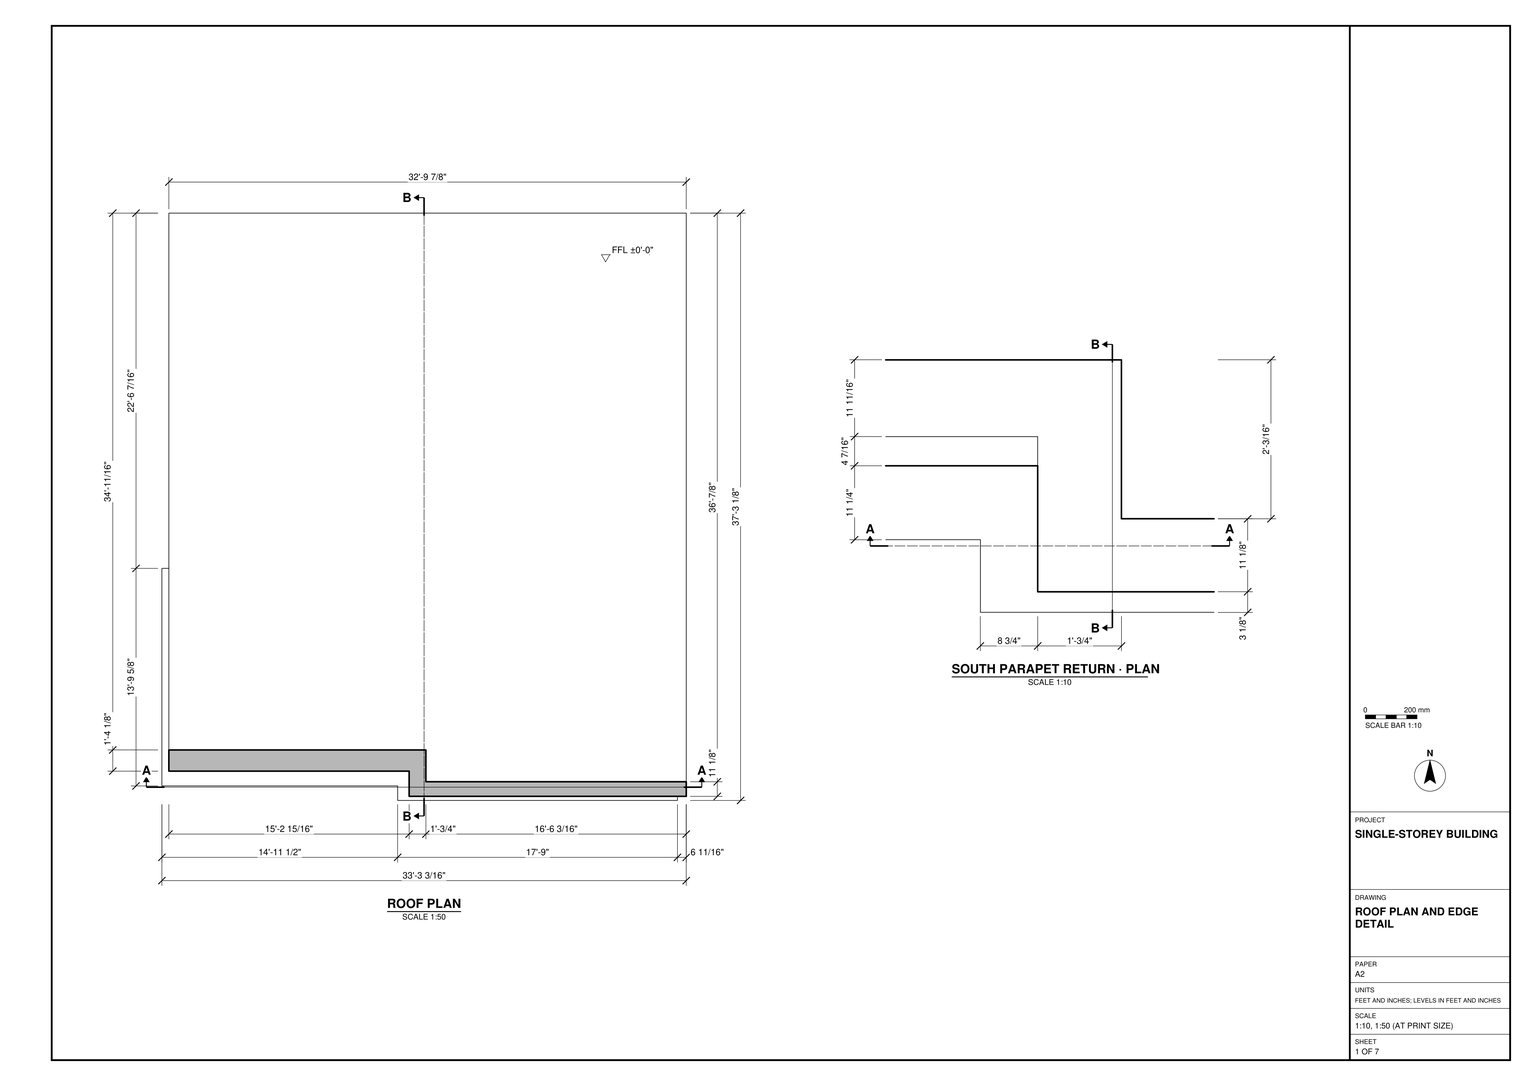
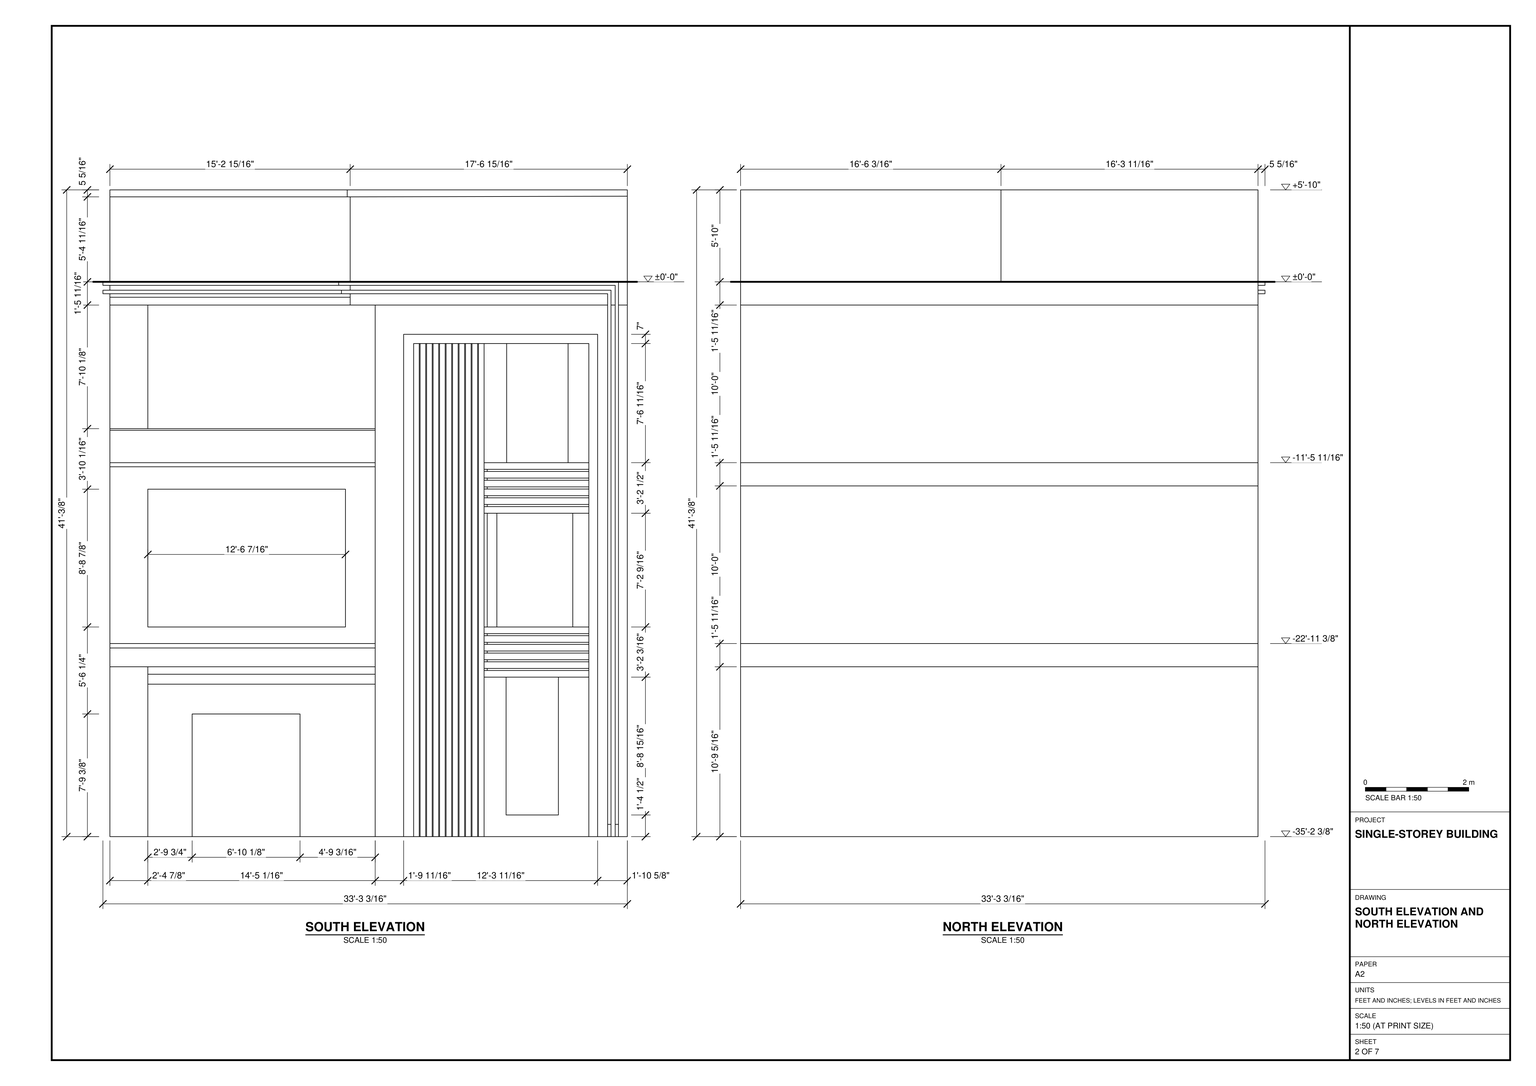
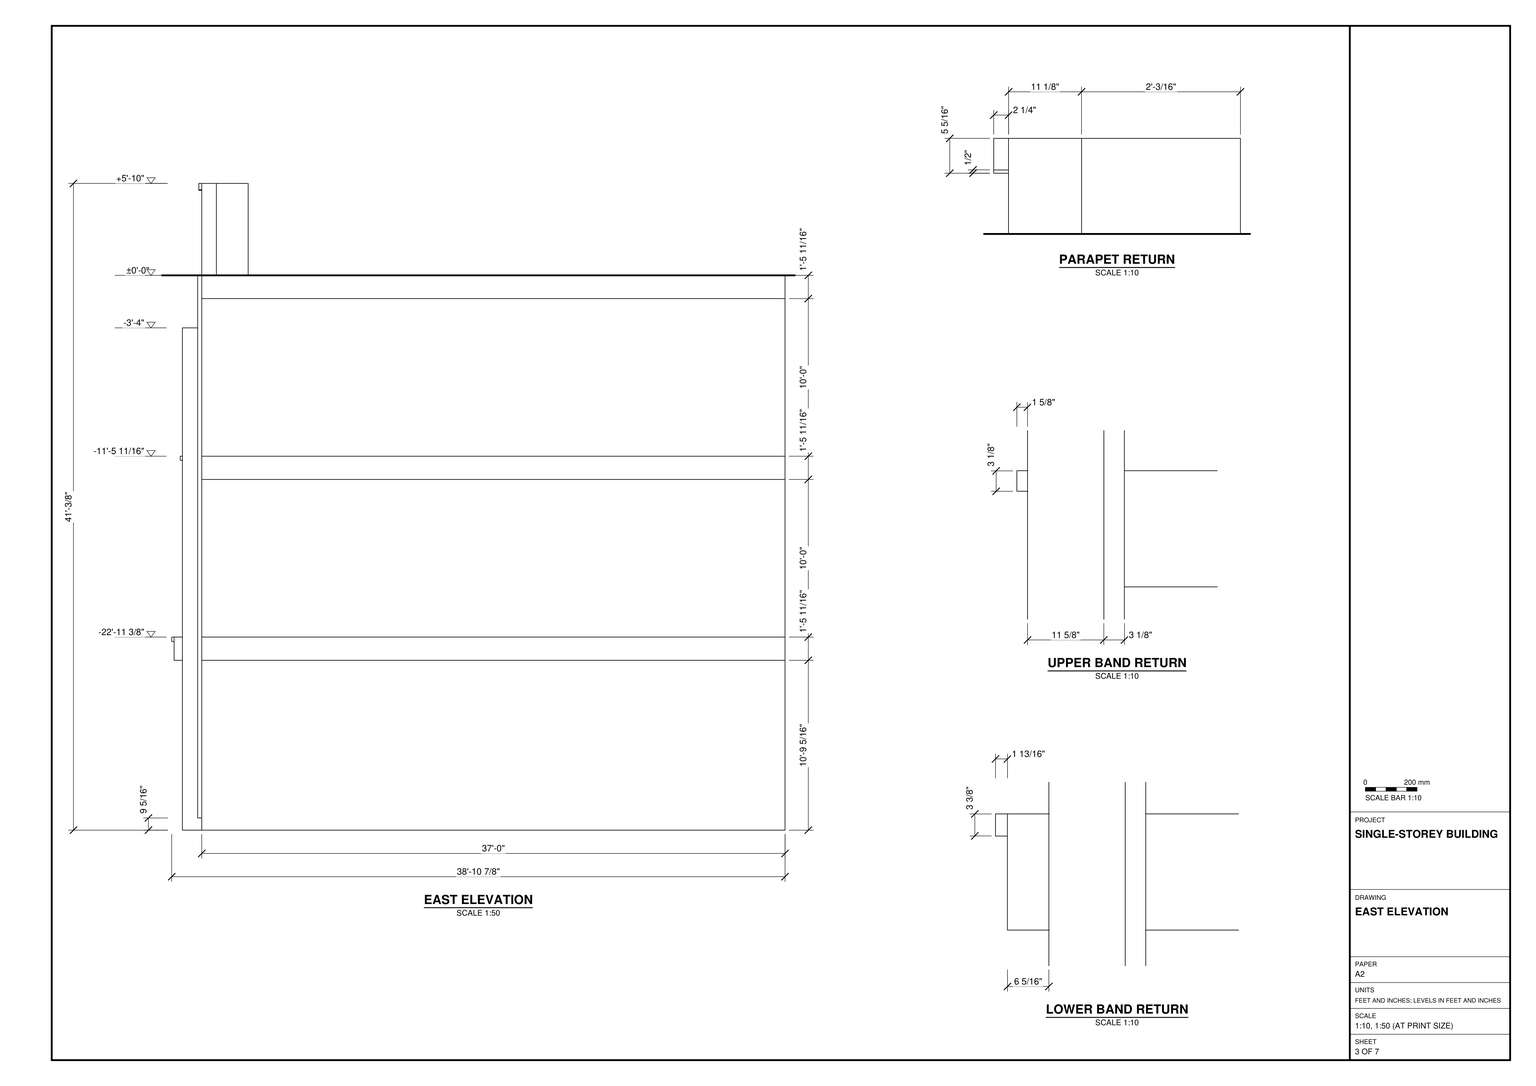
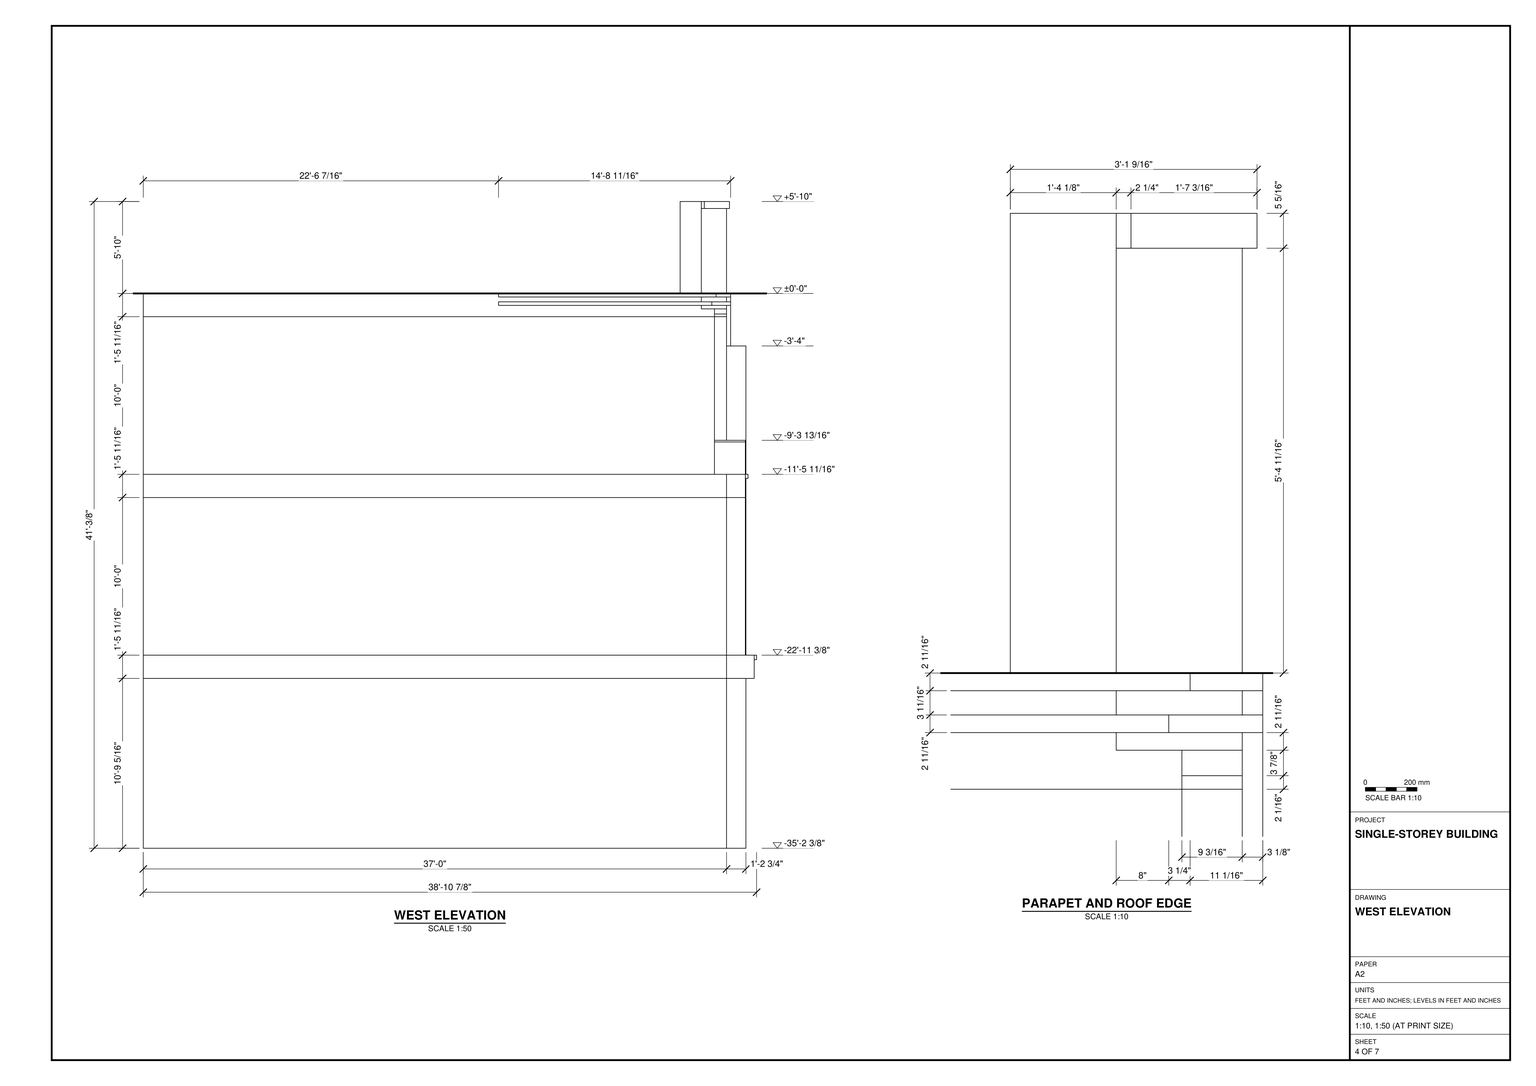
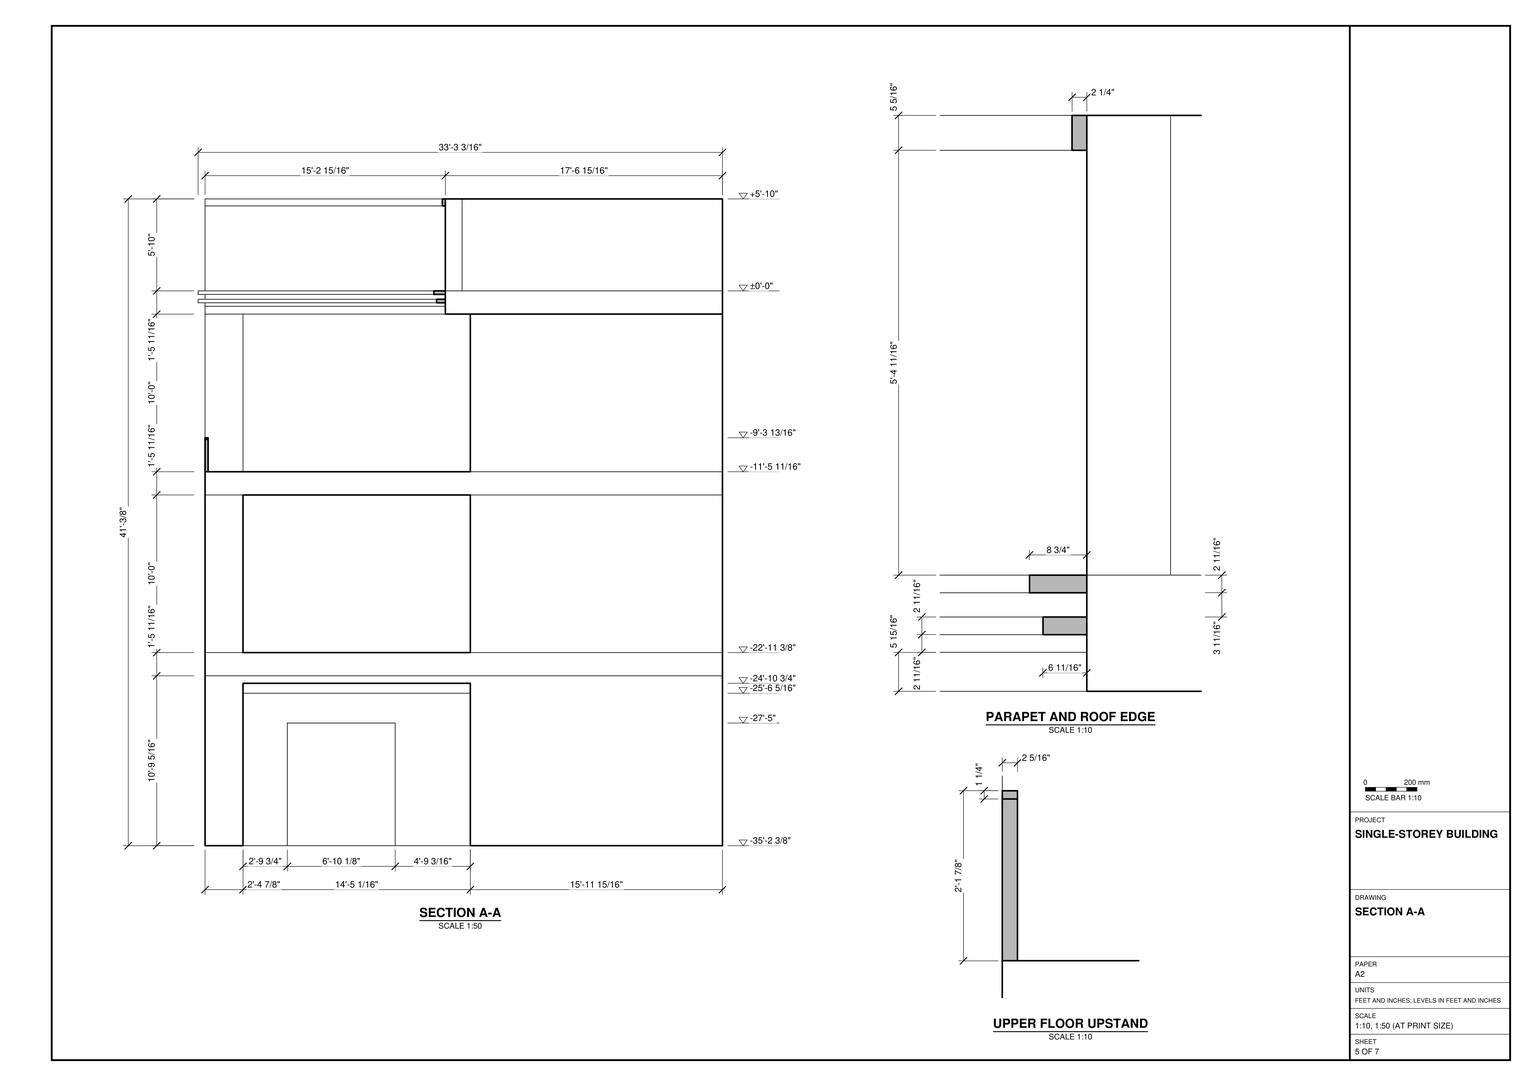
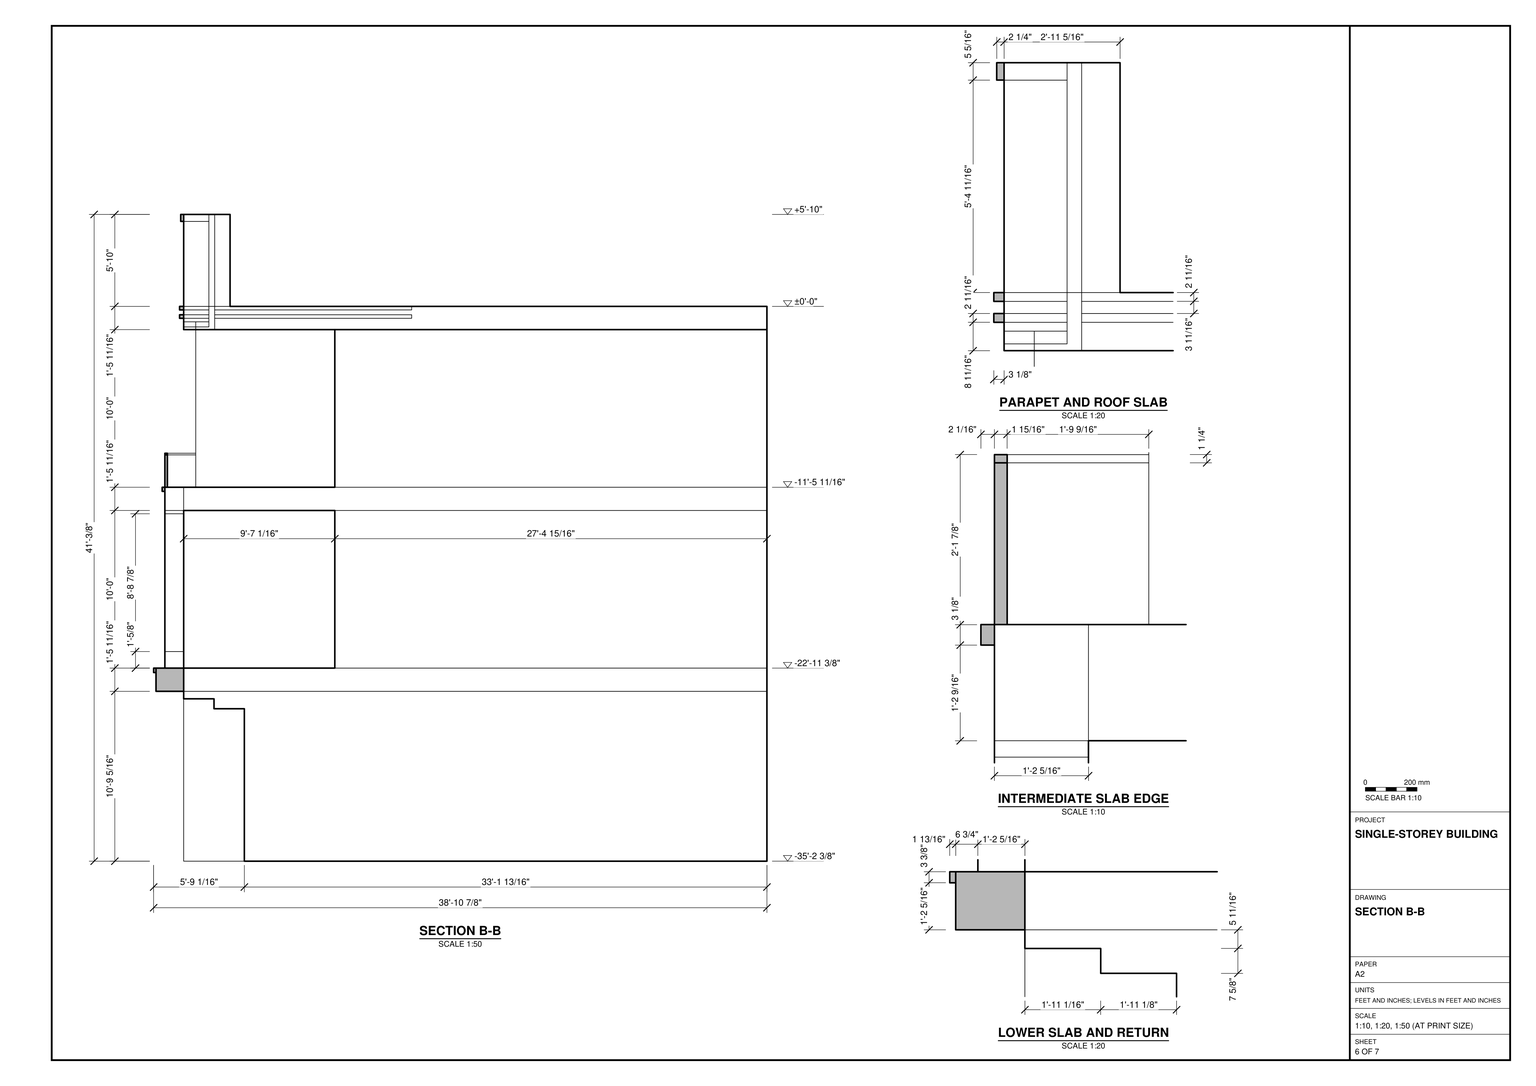
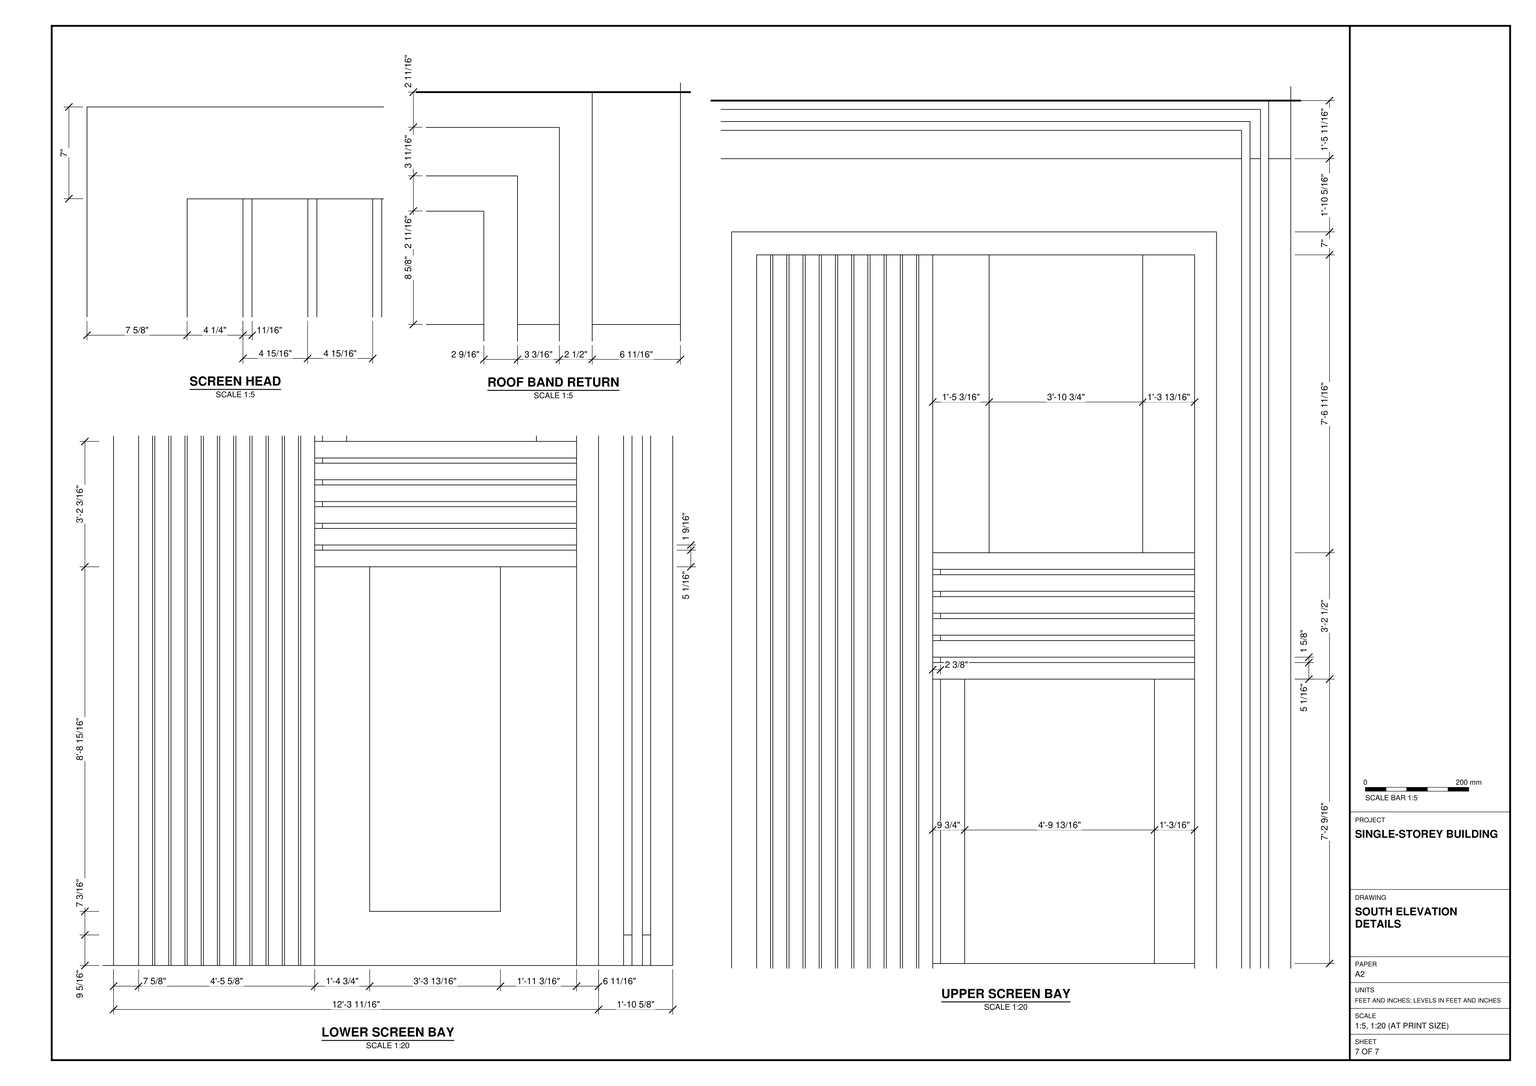
Build the exterior shell in SketchUp from task_files/diagram_01.pdf. Work in feet and inches. The overall dimensions, including projections, are 33'-3 3/16" east to west, 38'-10 7/8" north to south and 41'-3/8" high. Use the marked level ±0'-0" at the roof plane; the main wall faces extend below this datum and the south parapet rises above it.

Set out the walls and flat roof slab with the thicknesses shown. Follow the roof plan at the south edge, where a short return connects the two offset lengths of parapet. Use the elevations to align the slab edges and horizontal bands. On the south face, distinguish the broad left bay with its rectangular openings from the tall framed bay on the right. Within the frame, run the vertical fins alongside the stacked panels and horizontal slats. Use the edge details to give the bands, frame and parapet their drawn projections rather than representing them only with lines on a flat face.

Keep walls, slabs, roof and any furniture or joinery pieces shown in separate groups or components, and use components for repeated parts such as the fins. Any decor or loose items shown may use suitable library components. Save one SketchUp model as output_files/building_shell_with_stepped_parapet_and_screened_facade.skp.

# SketchUp Ruby script. Lengths in inches.
U = 1.inch
M = Sketchup.active_model
def pt(a) = Geom::Point3d.new(a.map { |v| v * U })
def face(e, loops, mat)
  f = e.add_face(loops[0].map { |a| pt(a) })
  loops[1..].each { |l| e.add_face(l.map { |a| pt(a) }).erase! }
  f.material = f.back_material = mat if mat
  f
end
# faces: each face lists its corners as indices into pts; further lists are holes
def faces(e, pts, list, mat = nil) = list.each { |f| face(e, (f[0].is_a?(Array) ? f : [f]).map { |l| l.map { |i| pts[i] } }, mat) }
# xy, xz, yz: faces in a plane at the given z, y or x. An outline is a flat list of corners, or four numbers for a rectangle; further outlines are holes
def ring(l) = l.size == 4 ? [[l[0], l[1]], [l[2], l[1]], [l[2], l[3]], [l[0], l[3]]] : l.each_slice(2).to_a
def flat(e, list, mat, &to3) = list.each { |f| face(e, (f[0].is_a?(Array) ? f : [f]).map { |l| ring(l).map { |u, v| to3.(u, v) } }, mat) }
def xy(e, z, list, mat = nil) = flat(e, list, mat) { |x, y| [x, y, z] }
def xz(e, y, list, mat = nil) = flat(e, list, mat) { |x, z| [x, y, z] }
def yz(e, x, list, mat = nil) = flat(e, list, mat) { |y, z| [x, y, z] }
def lines(e, pts, list) = list.each { |a, b| e.add_line(pt(pts[a]), pt(pts[b])) }
# prism: a flat outline (further loops are holes) pulled along v
def prism(e, loops, v, mat = nil)
  f = face(e, loops, mat); d = Geom::Vector3d.new(v.map { |x| x * U })
  f.pushpull(f.normal.samedirection?(d) ? d.length : -d.length)
end
def box(e, o, s, mat = nil) = prism(e, [[o, [o[0] + s[0], o[1], o[2]], [o[0] + s[0], o[1] + s[1], o[2]], [o[0], o[1] + s[1], o[2]]]], [0, 0, s[2]], mat)
def at(x, y, z, deg = 0) = Geom::Transformation.translation(pt([x, y, z])) * Geom::Transformation.rotation(ORIGIN, Z_AXIS, deg.degrees)
def axes(o, x, y, z) = Geom::Transformation.new([*x, 0, *y, 0, *z, 0, *pt(o).to_a, 1])
def part(name) = M.definitions.add(name)
# library, detail: a bought-in or finely detailed component or shape, given as its bounding box
def library(name, o, s) = part(name).tap { |d| box(d.entities, o, s) }
def detail(e, o, s) = box(e.add_group.entities, o, s)
def put(e, d, t, mat = nil) = e.add_instance(d, t).tap { |i| i.material = mat if mat }
def group(e, t, mat = nil) = e.add_group.tap { |g| g.transformation = t; g.material = mat if mat }.entities
root = M.entities
xy(root,-9.3125,[[228.91,8.125,228.91,22.875,207.25,22.875,207.25,69.0625,34.1875,69.0625,34.1875,22.875,5.3125,22.875,5.3125,466.875,399.1875,466.875,399.1875,22.875,376.59,22.875,376.59,8.125,369.9,8.125,369.9,22.875,290.16,22.875,290.16,18.625,285.91,18.625,285.91,22.875,285.22,22.875,285.22,18.625,280.97,18.625,280.97,22.875,280.29,22.875,280.29,18.625,276.04,18.625,276.04,22.875,275.35,22.875,275.35,18.625,271.1,18.625,271.1,22.875,270.41,22.875,270.41,18.625,266.16,18.625,266.16,22.875,265.47,22.875,265.47,18.625,261.22,18.625,261.22,22.875,260.54,22.875,260.54,18.625,256.29,18.625,256.29,22.875,255.6,22.875,255.6,18.625,251.35,18.625,251.35,22.875,250.66,22.875,250.66,18.625,246.41,18.625,246.41,22.875,245.72,22.875,245.72,18.625,241.47,18.625,241.47,22.875,240.79,22.875,240.79,18.625,236.54,18.625,236.54,8.125]])
xy(root,0,[[384.22,19.75,386.78,22.875],[389.97,19.75,392.47,22.875]])
xy(root,106.75,[[34.1875,45.97,207.25,69.0625]])
xy(root,112.11,[[290.16,16.125,369.9,22.875]])
xy(root,114.3125,[[34.1875,22.875,207.25,45.97]])
xy(root,117.17,[[290.16,16.125,369.9,22.875]])
xy(root,118.74,[[290.16,16.125,369.9,22.875]])
xy(root,120,[[5.3125,1.8125,34.1875,22.875],[34.1875,1.8125,207.25,22.875]])
xy(root,123.79,[[290.16,16.125,369.9,22.875]])
xy(root,125.36,[[290.16,16.125,369.9,22.875]])
xy(root,130.42,[[290.16,16.125,369.9,22.875]])
xy(root,131.99,[[290.16,16.125,369.9,22.875]])
xy(root,134.3125,[[5.3125,0,207.25,1.8125]])
xy(root,137.04,[[290.16,16.125,369.9,22.875]])
xy(root,137.6875,[[5.3125,0,207.25,1.8125],[5.3125,1.8125,207.25,8.5625],[5.3125,8.5625,34.1875,22.875],[34.1875,8.5625,207.25,22.875],[34.1875,22.875,207.25,137.9375]])
xy(root,138.61,[[290.16,16.125,369.9,22.875]])
xy(root,143.67,[[290.16,16.125,369.9,22.875]])
xy(root,145.24,[[290.16,17.375,369.9,22.875]])
xy(root,150.29,[[34.1875,8.5625,184.625,22.875],[290.16,17.375,369.9,22.875]])
xy(root,236.88,[[290.16,17.375,369.9,22.875]])
xy(root,241.9375,[[290.16,17.375,369.9,22.875]])
xy(root,243.57,[[290.16,17.375,369.9,22.875]])
xy(root,248.625,[[290.16,17.375,369.9,22.875]])
xy(root,250.26,[[290.16,17.375,369.9,22.875]])
xy(root,255.1875,[[34.1875,8.5625,184.625,22.875]])
xy(root,255.3125,[[290.16,17.375,369.9,22.875]])
xy(root,256.95,[[290.16,17.375,369.9,22.875]])
xy(root,257.6875,[[34.1875,22.875,207.25,137.9375]])
xy(root,262,[[290.16,17.375,369.9,22.875]])
xy(root,263.63,[[290.16,17.375,369.9,22.875]])
xy(root,268.6875,[[290.16,17.375,369.9,22.875]])
xy(root,270.32,[[290.16,17.375,369.9,22.875]])
xy(root,272.25,[[5.3125,6.5,207.25,8.5625]])
xy(root,275.375,[[5.3125,6.5,207.25,8.5625],[5.3125,8.5625,5.3125,32.0625,7.625,32.0625,7.625,10.5,207.25,10.5,207.25,8.5625],[7.625,10.5,207.25,10.5,207.25,22.875,34.1875,22.875,34.1875,32.0625,7.625,32.0625],[290.16,17.375,369.9,22.875],[34.1875,22.875,207.25,137.9375]])
xy(root,300,[[5.3125,8.5625,5.3125,32.0625,7.625,32.0625,7.625,10.5,207.25,10.5,207.25,8.5625]])
xy(root,301.25,[[5.3125,8.5625,207.25,8.5625,207.25,10.5,7.625,10.5,7.625,32.0625,5.3125,32.0625]])
xy(root,366.09,[[236.54,8.125,236.54,18.625,240.79,18.625,240.79,22.875,241.47,22.875,241.47,18.625,245.72,18.625,245.72,22.875,246.41,22.875,246.41,18.625,250.66,18.625,250.66,22.875,251.35,22.875,251.35,18.625,255.6,18.625,255.6,22.875,256.29,22.875,256.29,18.625,260.54,18.625,260.54,22.875,261.22,22.875,261.22,18.625,265.47,18.625,265.47,22.875,266.16,22.875,266.16,18.625,270.41,18.625,270.41,22.875,271.1,22.875,271.1,18.625,275.35,18.625,275.35,22.875,276.04,22.875,276.04,18.625,280.29,18.625,280.29,22.875,280.97,22.875,280.97,18.625,285.22,18.625,285.22,22.875,285.91,22.875,285.91,18.625,290.16,18.625,290.16,22.875,369.9,22.875,369.9,8.125]])
xy(root,373.09,[[228.91,8.125,376.59,22.875]])
xy(root,395.375,[[207.25,22.875,207.25,137.9375,34.1875,137.9375,34.1875,46.5,5.3125,46.5,5.3125,466.875,399.1875,466.875,399.1875,22.875],[188.22,22.875,188.22,46.5,34.1875,46.5,34.1875,137.9375,207.25,137.9375,207.25,22.875],[5.3125,32.0625,34.1875,46.5],[34.1875,32.0625,188.22,46.5]])
xy(root,401.3125,[[5.3125,32.0625,188.22,42.0625]])
xy(root,404,[[181.55,19.75,181.55,34.0625,0,34.0625,0,196.4375,5.3125,196.4375,5.3125,42.0625,188.22,42.0625,188.22,22.875,384.22,22.875,384.22,19.75]])
xy(root,406.6875,[[181.55,19.75,386.78,19.75,386.78,22.875,188.22,22.875,188.22,42.0625,5.3125,42.0625,5.3125,196.4375,0,196.4375,0,34.0625,181.55,34.0625]])
xy(root,410.375,[[179.5,19.75,179.5,30.8125,0,30.8125,0,196.4375,5.3125,196.4375,5.3125,42.0625,188.22,42.0625,188.22,22.875,389.97,22.875,389.97,19.75]])
xy(root,413.0625,[[179.5,19.75,392.47,19.75,392.47,22.875,188.22,22.875,188.22,42.0625,5.3125,42.0625,5.3125,196.4375,0,196.4375,0,30.8125,179.5,30.8125],[200.97,34,399.1875,34,399.1875,466.875,5.3125,466.875,5.3125,58.1875,200.97,58.1875],[5.3125,42.0625,188.22,46.5]])
xy(root,477.75,[[185.97,20.625,188.22,22.875],[185.97,22.875,185.97,39.8125,186.59,39.8125,186.59,42.0625,188.22,42.0625,188.22,22.875],[5.3125,39.8125,186.59,42.0625]])
xy(root,483.0625,[[185.97,20.625,399.1875,20.625,399.1875,22.875,188.22,22.875,188.22,42.0625,5.3125,42.0625,5.3125,39.8125,185.97,39.8125],[188.22,22.875,399.1875,22.875,399.1875,34,200.97,34,200.97,58.1875,5.3125,58.1875,5.3125,42.0625,188.22,42.0625]])
xz(root,0,[[5.3125,134.3125,207.25,137.6875]])
xz(root,1.8125,[[5.3125,120,207.25,134.3125],[5.3125,134.3125,207.25,137.6875]])
xz(root,6.5,[[5.3125,272.25,207.25,275.375]])
xz(root,8.125,[[228.91,-9.3125,236.54,-9.3125,236.54,366.09,369.9,366.09,369.9,-9.3125,376.59,-9.3125,376.59,373.09,228.91,373.09]])
xz(root,8.5625,[[[5.3125,137.6875,207.25,272.25],[34.1875,150.29,184.625,255.1875]],[5.3125,272.25,207.25,275.375],[5.3125,275.375,207.25,300],[5.3125,300,207.25,301.25]])
xz(root,10.5,[[7.625,275.375,207.25,300],[7.625,300,207.25,301.25]])
xz(root,16.125,[[290.16,112.11,369.9,117.17],[290.16,118.74,369.9,123.79],[290.16,125.36,369.9,130.42],[290.16,131.99,369.9,137.04],[290.16,138.61,369.9,143.67]])
xz(root,17.375,[[290.16,145.24,369.9,150.29],[290.16,236.88,369.9,241.9375],[290.16,243.57,369.9,248.625],[290.16,250.26,369.9,255.3125],[290.16,256.95,369.9,262],
  [290.16,263.63,369.9,268.6875],[290.16,270.32,369.9,275.375]])
xz(root,18.625,[[236.54,-9.3125,240.79,366.09],[241.47,-9.3125,245.72,366.09],[246.41,-9.3125,250.66,366.09],[251.35,-9.3125,255.6,366.09],[256.29,-9.3125,260.54,366.09],
  [261.22,-9.3125,265.47,366.09],[266.16,-9.3125,270.41,366.09],[271.1,-9.3125,275.35,366.09],[276.04,-9.3125,280.29,366.09],[280.97,-9.3125,285.22,366.09],
  [285.91,-9.3125,290.16,366.09]])
xz(root,19.75,[[389.97,0,392.47,0,392.47,413.0625,179.5,413.0625,179.5,410.375,389.97,410.375],[384.22,0,386.78,0,386.78,406.6875,181.55,406.6875,181.55,404,384.22,404]])
xz(root,20.625,[[185.97,477.75,188.22,477.75,399.1875,478.25,399.1875,483.0625,185.97,483.0625]])
xz(root,22.875,[[5.3125,-9.3125,34.1875,120],[207.25,-9.3125,228.91,-9.3125,228.91,373.09,376.59,373.09,376.59,-9.3125,384.22,-9.3125,384.22,395.375,207.25,395.375],[240.79,-9.3125,241.47,366.09],[245.72,-9.3125,246.41,366.09],[250.66,-9.3125,251.35,366.09],
  [255.6,-9.3125,256.29,366.09],[260.54,-9.3125,261.22,366.09],[265.47,-9.3125,266.16,366.09],[270.41,-9.3125,271.1,366.09],[275.35,-9.3125,276.04,366.09],
  [280.29,-9.3125,280.97,366.09],[285.22,-9.3125,285.91,366.09],[290.16,-9.3125,369.9,-9.3125,369.9,112.11,346.72,112.11,346.72,7.18,306.91,7.18,306.91,112.11,290.16,112.11],[384.22,-9.3125,386.78,0],[386.78,-9.3125,389.97,395.375],
  [389.97,-9.3125,392.47,0],[392.47,-9.3125,399.1875,395.375],[384.22,0,386.78,395.375],[389.97,0,392.47,395.375],[306.91,7.18,346.72,112.11],
  [34.1875,114.3125,207.25,120],[290.16,117.17,292.54,118.74],[292.54,117.17,369.9,118.74],[5.3125,120,207.25,137.6875],[290.16,123.79,292.54,125.36],
  [292.54,123.79,369.9,125.36],[290.16,130.42,292.54,131.99],[292.54,130.42,369.9,131.99],[290.16,137.04,292.54,138.61],[292.54,137.04,369.9,138.61],
  [5.3125,137.6875,34.1875,257.6875],[34.1875,137.6875,34.1875,150.29,184.625,150.29,184.625,255.1875,195.3125,255.1875,195.3125,257.6875,207.25,257.6875,207.25,137.6875],[290.16,143.67,292.54,145.24],[292.54,143.67,369.9,145.24],[290.16,150.29,292.54,236.88],
  [292.54,150.29,299.89,236.88],[299.89,150.29,357.68,236.88],[357.68,150.29,369.9,236.88],[290.16,241.9375,292.54,243.57],[292.54,241.9375,369.9,243.57],
  [290.16,248.625,292.54,250.26],[292.54,248.625,369.9,250.26],[34.1875,255.1875,195.3125,257.6875],[290.16,255.3125,292.54,256.95],[292.54,255.3125,369.9,256.95],
  [290.16,262,292.54,263.63],[292.54,262,369.9,263.63],[290.16,268.6875,292.54,270.32],[292.54,268.6875,369.9,270.32],[290.16,275.375,307.35,366.09],
  [307.35,275.375,354.11,366.09],[354.11,275.375,369.9,366.09],[188.22,395.375,384.22,404],[384.22,395.375,386.78,395.375,386.78,406.6875,188.22,406.6875,188.22,404,384.22,404],[386.78,395.375,389.97,395.375,389.97,410.375,188.22,410.375,188.22,406.6875,386.78,406.6875],
  [389.97,395.375,392.47,395.375,392.47,413.0625,188.22,413.0625,188.22,410.375,389.97,410.375],[392.47,395.375,399.1875,395.375,399.1875,478.25,188.22,477.75,188.22,413.0625,392.47,413.0625],[188.22,477.75,188.22,483.0625,399.1875,483.0625,399.1875,478.25]])
xz(root,30.8125,[[0,410.375,179.5,413.0625]])
xz(root,32.0625,[[7.625,275.375,34.1875,275.375,34.1875,395.375,5.3125,395.375,5.3125,301.25,7.625,301.25],[5.3125,395.375,188.22,401.3125]])
xz(root,34,[[200.97,413.0625,399.1875,483.0625]])
xz(root,34.0625,[[0,404,181.55,406.6875]])
xz(root,39.8125,[[5.3125,477.75,185.97,483.0625]])
xz(root,42.0625,[[5.3125,401.3125,188.22,404],[5.3125,404,188.22,406.6875],[5.3125,406.6875,188.22,410.375],[5.3125,410.375,188.22,413.0625],[5.3125,413.0625,188.22,477.75],
  [5.3125,477.75,186.59,483.0625],[186.59,477.75,188.22,483.0625]])
xz(root,45.97,[[34.1875,106.75,207.25,114.3125]])
xz(root,58.1875,[[5.3125,413.0625,200.97,483.0625]])
xz(root,69.0625,[[34.1875,-9.3125,67.93,-9.3125,67.93,84.0625,150.05,84.0625,150.05,-9.3125,207.25,-9.3125,207.25,106.75,34.1875,106.75],[67.93,-9.3125,150.05,84.0625]])
xz(root,137.9375,[[34.1875,137.6875,207.25,257.6875],[34.1875,275.375,207.25,395.375]])
xz(root,196.4375,[[0,404,5.3125,406.6875],[0,410.375,5.3125,413.0625]])
xz(root,466.875,[[5.3125,-9.3125,399.1875,120],[5.3125,120,399.1875,137.6875],[5.3125,137.6875,399.1875,257.6875],[5.3125,257.6875,399.1875,275.375],[5.3125,275.375,399.1875,395.375],
  [5.3125,395.375,399.1875,413.0625]])
yz(root,0,[[34.0625,404,196.4375,406.6875],[30.8125,410.375,196.4375,413.0625]])
yz(root,5.3125,[[22.875,-9.3125,466.875,120],[1.8125,120,22.875,137.6875],[22.875,120,466.875,137.6875],[0,134.3125,1.8125,137.6875],[8.5625,137.6875,22.875,257.6875],
  [22.875,137.6875,466.875,257.6875],[8.5625,257.6875,22.875,275.375],[22.875,257.6875,466.875,275.375],[6.5,272.25,8.5625,275.375],[8.5625,275.375,32.0625,300],
  [32.0625,275.375,466.875,395.375],[8.5625,300,32.0625,301.25],[32.0625,395.375,32.0625,401.3125,42.0625,401.3125,42.0625,404,196.4375,404,196.4375,406.6875,42.0625,406.6875,42.0625,410.375,196.4375,410.375,196.4375,413.0625,466.875,413.0625,466.875,395.375],[42.0625,404,196.4375,406.6875],[42.0625,410.375,196.4375,413.0625],
  [42.0625,413.0625,58.1875,483.0625],[39.8125,477.75,42.0625,483.0625]])
yz(root,7.625,[[10.5,275.375,32.0625,300],[10.5,300,32.0625,301.25]])
yz(root,34.1875,[[22.875,-9.3125,69.0625,-9.3125,69.0625,106.75,45.97,106.75,45.97,114.3125,22.875,114.3125],[22.875,137.6875,137.9375,257.6875],[8.5625,150.29,22.875,255.1875],[32.0625,275.375,137.9375,395.375]])
yz(root,179.5,[[19.75,410.375,30.8125,413.0625]])
yz(root,181.55,[[19.75,404,34.0625,406.6875]])
yz(root,184.625,[[8.5625,150.29,22.875,255.1875]])
yz(root,185.97,[[20.625,477.75,39.8125,483.0625]])
yz(root,188.22,[[22.875,395.375,32.0625,397.4375],[32.0625,395.375,32.0625,397.4375,42.0625,397.4375,42.0625,413.0625,46.5,413.0625,46.5,395.375],[22.875,397.4375,32.0625,401.3125],[32.0625,397.4375,42.0625,401.3125],[22.875,401.3125,42.0625,404],
  [22.875,404,42.0625,406.6875],[22.875,406.6875,42.0625,410.375],[22.875,410.375,42.0625,413.0625],[22.875,413.0625,42.0625,477.75],[22.875,477.75,42.0625,483.0625]])
yz(root,200.97,[[34,413.0625,58.1875,483.0625]])
yz(root,207.25,[[22.875,-9.3125,22.875,114.3125,45.97,114.3125,45.97,106.75,69.0625,106.75,69.0625,-9.3125],[1.8125,120,22.875,137.6875],[0,134.3125,1.8125,137.6875],[8.5625,137.6875,22.875,257.6875],[22.875,137.6875,137.9375,257.6875],
  [8.5625,257.6875,22.875,275.375],[6.5,272.25,8.5625,275.375],[8.5625,275.375,10.5,300],[22.875,275.375,137.9375,395.375],[8.5625,300,10.5,301.25]])
yz(root,228.91,[[8.125,-9.3125,22.875,373.09]])
yz(root,236.54,[[8.125,-9.3125,18.625,366.09]])
yz(root,240.79,[[18.625,-9.3125,22.875,366.09]])
yz(root,241.47,[[18.625,-9.3125,22.875,366.09]])
yz(root,245.72,[[18.625,-9.3125,22.875,366.09]])
yz(root,246.41,[[18.625,-9.3125,22.875,366.09]])
yz(root,250.66,[[18.625,-9.3125,22.875,366.09]])
yz(root,251.35,[[18.625,-9.3125,22.875,366.09]])
yz(root,255.6,[[18.625,-9.3125,22.875,366.09]])
yz(root,256.29,[[18.625,-9.3125,22.875,366.09]])
yz(root,260.54,[[18.625,-9.3125,22.875,366.09]])
yz(root,261.22,[[18.625,-9.3125,22.875,366.09]])
yz(root,265.47,[[18.625,-9.3125,22.875,366.09]])
yz(root,266.16,[[18.625,-9.3125,22.875,366.09]])
yz(root,270.41,[[18.625,-9.3125,22.875,366.09]])
yz(root,271.1,[[18.625,-9.3125,22.875,366.09]])
yz(root,275.35,[[18.625,-9.3125,22.875,366.09]])
yz(root,276.04,[[18.625,-9.3125,22.875,366.09]])
yz(root,280.29,[[18.625,-9.3125,22.875,366.09]])
yz(root,280.97,[[18.625,-9.3125,22.875,366.09]])
yz(root,285.22,[[18.625,-9.3125,22.875,366.09]])
yz(root,285.91,[[18.625,-9.3125,22.875,366.09]])
yz(root,290.16,[[18.625,-9.3125,22.875,112.11],[16.125,112.11,18.625,117.17],[18.625,112.11,22.875,117.17],[18.625,117.17,22.875,118.74],[16.125,118.74,18.625,123.79],
  [18.625,118.74,22.875,123.79],[18.625,123.79,22.875,125.36],[16.125,125.36,18.625,130.42],[18.625,125.36,22.875,130.42],[18.625,130.42,22.875,131.99],
  [16.125,131.99,18.625,137.04],[18.625,131.99,22.875,137.04],[18.625,137.04,22.875,138.61],[16.125,138.61,18.625,143.67],[18.625,138.61,22.875,143.67],
  [18.625,143.67,22.875,145.24],[17.375,145.24,18.625,150.29],[18.625,145.24,22.875,150.29],[18.625,150.29,22.875,236.88],[17.375,236.88,18.625,241.9375],
  [18.625,236.88,22.875,241.9375],[18.625,241.9375,22.875,243.57],[17.375,243.57,18.625,248.625],[18.625,243.57,22.875,248.625],[18.625,248.625,22.875,250.26],
  [17.375,250.26,18.625,255.3125],[18.625,250.26,22.875,255.3125],[18.625,255.3125,22.875,256.95],[17.375,256.95,18.625,262],[18.625,256.95,22.875,262],
  [18.625,262,22.875,263.63],[17.375,263.63,18.625,268.6875],[18.625,263.63,22.875,268.6875],[18.625,268.6875,22.875,270.32],[17.375,270.32,18.625,275.375],
  [18.625,270.32,22.875,275.375],[18.625,275.375,22.875,366.09]])
yz(root,369.9,[[8.125,-9.3125,8.125,120,16.125,120,16.125,118.74,22.875,118.74,22.875,117.17,16.125,117.17,16.125,112.11,22.875,112.11,22.875,-9.3125],[8.125,120,8.125,137.6875,22.875,137.6875,22.875,137.04,16.125,137.04,16.125,131.99,22.875,131.99,22.875,130.42,16.125,130.42,16.125,125.36,22.875,125.36,22.875,123.79,16.125,123.79,16.125,120],[8.125,137.6875,8.125,257.6875,17.375,257.6875,17.375,256.95,22.875,256.95,22.875,255.3125,17.375,255.3125,17.375,250.26,22.875,250.26,22.875,248.625,17.375,248.625,17.375,243.57,22.875,243.57,22.875,241.9375,17.375,241.9375,17.375,236.88,22.875,236.88,22.875,150.29,17.375,150.29,17.375,145.24,22.875,145.24,22.875,143.67,16.125,143.67,16.125,138.61,22.875,138.61,22.875,137.6875],[8.125,257.6875,8.125,275.375,17.375,275.375,17.375,270.32,22.875,270.32,22.875,268.6875,17.375,268.6875,17.375,263.63,22.875,263.63,22.875,262,17.375,262,17.375,257.6875],[8.125,275.375,22.875,366.09]])
yz(root,376.59,[[8.125,-9.3125,22.875,373.09]])
yz(root,384.22,[[19.75,0,22.875,404]])
yz(root,386.78,[[19.75,0,22.875,406.6875]])
yz(root,389.97,[[19.75,0,22.875,410.375]])
yz(root,392.47,[[19.75,0,22.875,413.0625]])
yz(root,399.1875,[[22.875,-9.3125,466.875,120],[22.875,120,466.875,137.6875],[22.875,137.6875,466.875,257.6875],[22.875,257.6875,466.875,275.375],[22.875,275.375,466.875,395.375],
  [22.875,395.375,466.875,395.375,466.875,413.0625,34,413.0625,34,483.0625,22.875,483.0625],[20.625,478.25,22.875,483.0625]])
p = [[188.22,22.875,477.75],[399.1875,22.875,478.25],[399.1875,20.625,478.25],[188.22,20.625,477.75],[188.22,46.5,413.0625],[188.22,46.5,483.0625],
  [34.1875,22.875,257.6875],[34.1875,8.5625,257.6875],[5.3125,42.0625,397.4375],[188.22,42.0625,397.4375]]
faces(root,p,[[0,1,2,3]])
lines(root,p,[[4,5],[6,7],[8,9]])
